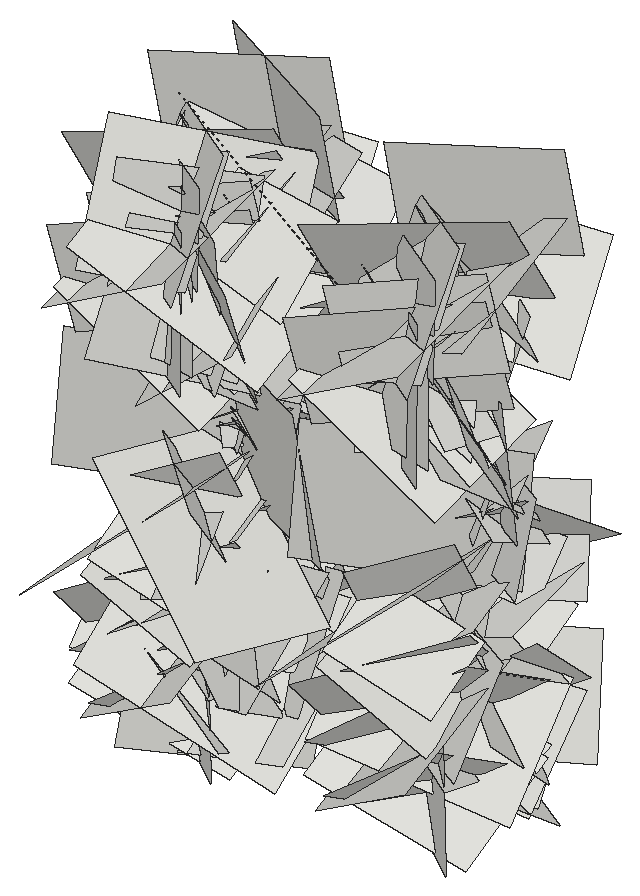
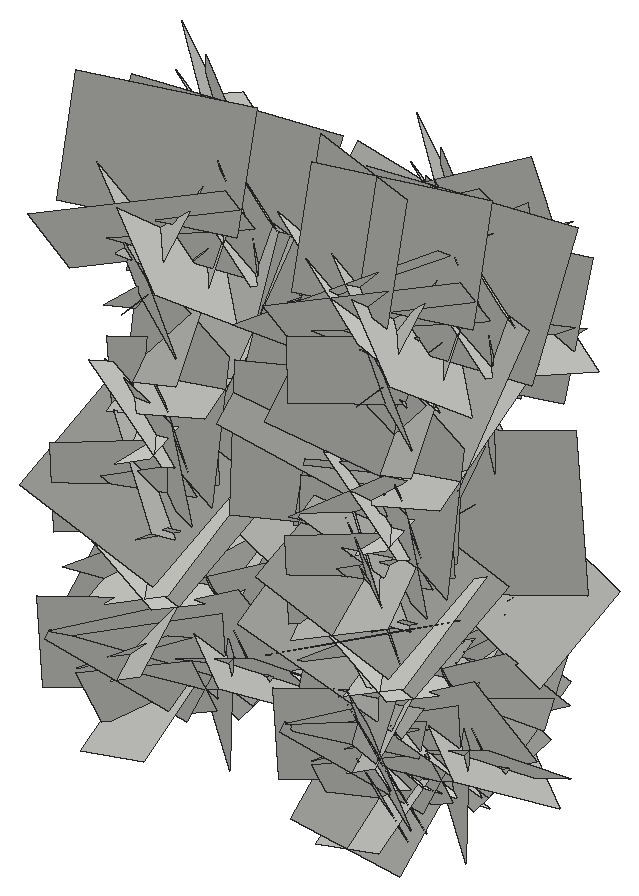
# SketchUp Ruby script. Lengths in inches.
U = 1.inch
M = Sketchup.active_model
def pt(a) = Geom::Point3d.new(a.map { |v| v * U })
def face(e, loops, mat)
  f = e.add_face(loops[0].map { |a| pt(a) })
  loops[1..].each { |l| e.add_face(l.map { |a| pt(a) }).erase! }
  f.material = f.back_material = mat if mat
  f
end
# faces: each face lists its corners as indices into pts; further lists are holes
def faces(e, pts, list, mat = nil) = list.each { |f| face(e, (f[0].is_a?(Array) ? f : [f]).map { |l| l.map { |i| pts[i] } }, mat) }
# xy, xz, yz: faces in a plane at the given z, y or x. An outline is a flat list of corners, or four numbers for a rectangle; further outlines are holes
def ring(l) = l.size == 4 ? [[l[0], l[1]], [l[2], l[1]], [l[2], l[3]], [l[0], l[3]]] : l.each_slice(2).to_a
def flat(e, list, mat, &to3) = list.each { |f| face(e, (f[0].is_a?(Array) ? f : [f]).map { |l| ring(l).map { |u, v| to3.(u, v) } }, mat) }
def xy(e, z, list, mat = nil) = flat(e, list, mat) { |x, y| [x, y, z] }
def xz(e, y, list, mat = nil) = flat(e, list, mat) { |x, z| [x, y, z] }
def yz(e, x, list, mat = nil) = flat(e, list, mat) { |y, z| [x, y, z] }
def lines(e, pts, list) = list.each { |a, b| e.add_line(pt(pts[a]), pt(pts[b])) }
# prism: a flat outline (further loops are holes) pulled along v
def prism(e, loops, v, mat = nil)
  f = face(e, loops, mat); d = Geom::Vector3d.new(v.map { |x| x * U })
  f.pushpull(f.normal.samedirection?(d) ? d.length : -d.length)
end
def box(e, o, s, mat = nil) = prism(e, [[o, [o[0] + s[0], o[1], o[2]], [o[0] + s[0], o[1] + s[1], o[2]], [o[0], o[1] + s[1], o[2]]]], [0, 0, s[2]], mat)
def at(x, y, z, deg = 0) = Geom::Transformation.translation(pt([x, y, z])) * Geom::Transformation.rotation(ORIGIN, Z_AXIS, deg.degrees)
def axes(o, x, y, z) = Geom::Transformation.new([*x, 0, *y, 0, *z, 0, *pt(o).to_a, 1])
def part(name) = M.definitions.add(name)
# library, detail: a bought-in or finely detailed component or shape, given as its bounding box
def library(name, o, s) = part(name).tap { |d| box(d.entities, o, s) }
def detail(e, o, s) = box(e.add_group.entities, o, s)
def put(e, d, t, mat = nil) = e.add_instance(d, t).tap { |i| i.material = mat if mat }
def group(e, t, mat = nil) = e.add_group.tap { |g| g.transformation = t; g.material = mat if mat }.entities
root = M.entities
c1 = part("Component\#6")
p = [[0.01,0,0],[0,3.24,4.54],[4.32,3.24,4.54],[4.33,0,0]]
faces(c1.entities,p,[[0,1,2,3]])
put(root,c1,axes([404.88,204.41,7.91],[-0.10208,-0.52254,-0.48763],[-0.08086,-0.48171,0.53127],[-0.75328,0.12252,0.00905]))
put(root,c1,axes([400.91,204.41,7.91],[0.10208,-0.52254,-0.48763],[0.08086,-0.48171,0.53127],[0.75328,0.12252,0.00905]))
put(root,c1,axes([414.68,204.41,7.91],[-0.10208,-0.52254,-0.48763],[-0.08086,-0.48171,0.53127],[-0.75328,0.12252,0.00905]))
put(root,c1,axes([400.91,200.61,7.25],[-0.15258,0.77944,0.1154],[-0.02035,0.1138,-0.79262],[0.83497,0.14521,0.00177]))
put(root,c1,axes([404.88,200.61,7.25],[0.15258,0.77944,0.1154],[0.02035,0.1138,-0.79262],[-0.83497,0.14521,0.00177]))
put(root,c1,axes([410.71,200.61,7.25],[-0.15258,0.77944,0.1154],[-0.02035,0.1138,-0.79262],[0.83497,0.14521,0.00177]))
put(root,c1,axes([404.88,201.43,15.61],[-0.13511,0.17275,0.7909],[-0.07376,0.79534,-0.18493],[-0.85494,-0.09592,-0.10904]))
put(root,c1,axes([400.91,201.43,15.61],[0.13511,0.17275,0.7909],[0.07376,0.79534,-0.18493],[0.85494,-0.09592,-0.10904]))
put(root,c1,axes([414.68,201.43,15.61],[-0.13511,0.17275,0.7909],[-0.07376,0.79534,-0.18493],[-0.85494,-0.09592,-0.10904]))
put(root,c1,axes([404.88,201.2,11.35],[-0.2643,1.29708,-0.17492],[0.19217,-0.14212,-1.31229],[-1.37397,-0.26938,-0.1499]))
put(root,c1,axes([400.91,201.2,11.35],[0.2643,1.29708,-0.17492],[-0.19217,-0.14212,-1.31229],[1.37397,-0.26938,-0.1499]))
put(root,c1,axes([414.68,201.2,11.35],[-0.2643,1.29708,-0.17492],[0.19217,-0.14212,-1.31229],[-1.37397,-0.26938,-0.1499]))
put(root,c1,axes([404.88,201.6875,18.6875],[-0.06388,0.10125,0.82658],[0.05301,0.82768,-0.09774],[-0.88113,0.04245,-0.0658]))
put(root,c1,axes([400.91,201.6875,18.6875],[0.06388,0.10125,0.82658],[-0.05301,0.82768,-0.09774],[0.88113,0.04245,-0.0658]))
put(root,c1,axes([414.68,201.6875,18.6875],[-0.06388,0.10125,0.82658],[0.05301,0.82768,-0.09774],[-0.88113,0.04245,-0.0658]))
put(root,c1,axes([404.88,204.39,20.61],[-0.01972,0.37325,-1.09096],[-0.03348,-1.09086,-0.37268],[-1.22177,0.02387,0.02782]))
put(root,c1,axes([400.91,204.39,20.61],[0.01972,0.37325,-1.09096],[0.03348,-1.09086,-0.37268],[1.22177,0.02387,0.02782]))
put(root,c1,axes([414.68,204.39,20.61],[-0.01972,0.37325,-1.09096],[-0.03348,-1.09086,-0.37268],[-1.22177,0.02387,0.02782]))
put(root,c1,axes([404.88,199.86,19.8],[0.08167,1.25653,0.46028],[-0.00634,0.46136,-1.25848],[-1.41846,0.07029,0.03212]))
put(root,c1,axes([400.91,199.86,19.8],[-0.08167,1.25653,0.46028],[0.00634,0.46136,-1.25848],[1.41846,0.07029,0.03212]))
put(root,c1,axes([414.68,199.86,19.8],[0.08167,1.25653,0.46028],[-0.00634,0.46136,-1.25848],[-1.41846,0.07029,0.03212]))
put(root,c1,axes([400.91,203.18,8],[0.06036,-0.35202,0.5516],[-0.07606,0.54699,0.35648],[0.68943,0.09116,-0.00896]))
put(root,c1,axes([404.88,203.18,8],[-0.06036,-0.35202,0.5516],[0.07606,0.54699,0.35648],[-0.68943,0.09116,-0.00896]))
put(root,c1,axes([410.71,203.18,8],[0.06036,-0.35202,0.5516],[-0.07606,0.54699,0.35648],[0.68943,0.09116,-0.00896]))
put(root,c1,axes([404.88,204.45,21.63],[0.07523,0.18922,-0.91056],[-0.04715,-0.91147,-0.19287],[-0.98469,0.0581,-0.06033]))
put(root,c1,axes([400.91,204.45,21.63],[-0.07523,0.18922,-0.91056],[0.04715,-0.91147,-0.19287],[0.98469,0.0581,-0.06033]))
put(root,c1,axes([414.68,204.45,21.63],[0.07523,0.18922,-0.91056],[-0.04715,-0.91147,-0.19287],[-0.98469,0.0581,-0.06033]))
put(root,c1,axes([404.88,203.64,8.5],[-0.20575,0.76434,-0.74551],[0.06488,-0.74852,-0.78336],[-1.12991,-0.18216,0.09078]))
put(root,c1,axes([400.91,203.64,8.5],[0.20575,0.76434,-0.74551],[-0.06488,-0.74852,-0.78336],[1.12991,-0.18216,0.09078]))
put(root,c1,axes([414.68,203.64,8.5],[-0.20575,0.76434,-0.74551],[0.06488,-0.74852,-0.78336],[-1.12991,-0.18216,0.09078]))
put(root,c1,axes([404.88,201.07,18.92],[-0.13602,0.69446,0.8684],[-0.06726,0.86816,-0.70365],[-1.17673,-0.1299,-0.06016]))
put(root,c1,axes([400.91,201.07,18.92],[0.13602,0.69446,0.8684],[0.06726,0.86816,-0.70365],[1.17673,-0.1299,-0.06016]))
put(root,c1,axes([414.68,201.07,18.92],[-0.13602,0.69446,0.8684],[-0.06726,0.86816,-0.70365],[-1.17673,-0.1299,-0.06016]))
put(root,c1,axes([404.88,200.34,18.7],[0.08817,0.51183,1.11442],[0.20058,1.09825,-0.51853],[-1.28435,0.20665,-0.00447]))
put(root,c1,axes([400.91,200.34,18.7],[-0.08817,0.51183,1.11442],[-0.20058,1.09825,-0.51853],[1.28435,0.20665,-0.00447]))
put(root,c1,axes([414.68,200.34,18.7],[0.08817,0.51183,1.11442],[0.20058,1.09825,-0.51853],[-1.28435,0.20665,-0.00447]))
put(root,c1,axes([404.88,200.79,15.19],[-0.21334,0.28139,1.2169],[0.22593,1.22225,-0.24738],[-1.30453,0.16566,-0.24185]))
put(root,c1,axes([400.91,200.79,15.19],[0.21334,0.28139,1.2169],[-0.22593,1.22225,-0.24738],[1.30453,0.16566,-0.24185]))
put(root,c1,axes([414.68,200.79,15.19],[-0.21334,0.28139,1.2169],[0.22593,1.22225,-0.24738],[-1.30453,0.16566,-0.24185]))
put(root,c1,axes([400.91,205.06,0.06],[-0.16762,-0.72435,0.3647],[-0.00744,0.37278,0.73735],[0.85961,-0.13802,0.0775]))
put(root,c1,axes([404.88,205.06,0.06],[0.16762,-0.72435,0.3647],[0.00744,0.37278,0.73735],[-0.85961,-0.13802,0.0775]))
put(root,c1,axes([410.71,205.06,0.06],[-0.16762,-0.72435,0.3647],[-0.00744,0.37278,0.73735],[0.85961,-0.13802,0.0775]))
put(root,c1,axes([400.91,202.62,14.39],[-0.09007,0.1944,0.61889],[0.03503,0.62466,-0.19168],[0.68673,-0.00637,0.09095]))
put(root,c1,axes([404.88,202.62,14.39],[0.09007,0.1944,0.61889],[-0.03503,0.62466,-0.19168],[-0.68673,-0.00637,0.09095]))
put(root,c1,axes([410.71,202.62,14.39],[-0.09007,0.1944,0.61889],[0.03503,0.62466,-0.19168],[0.68673,-0.00637,0.09095]))
put(root,c1,axes([404.88,200.25,4.04],[0.10038,1.14624,0.70824],[0.13093,0.69961,-1.1488],[-1.42222,0.14531,-0.05578]))
put(root,c1,axes([400.91,200.25,4.04],[-0.10038,1.14624,0.70824],[-0.13093,0.69961,-1.1488],[1.42222,0.14531,-0.05578]))
put(root,c1,axes([414.68,200.25,4.04],[0.10038,1.14624,0.70824],[0.13093,0.69961,-1.1488],[-1.42222,0.14531,-0.05578]))
put(root,c1,axes([404.88,207.09,15.04],[-0.15807,-1.02909,-0.4958],[0.14338,-0.5124,1.02286],[-1.20232,0.07419,0.18716]))
put(root,c1,axes([400.91,207.09,15.04],[0.15807,-1.02909,-0.4958],[-0.14338,-0.5124,1.02286],[1.20232,0.07419,0.18716]))
put(root,c1,axes([414.68,207.09,15.04],[-0.15807,-1.02909,-0.4958],[0.14338,-0.5124,1.02286],[-1.20232,0.07419,0.18716]))
put(root,c1,axes([400.91,205.68,16.84],[0.07036,-0.63328,-0.02287],[-0.09357,-0.03201,0.6302],[0.66517,0.06248,0.09107]))
put(root,c1,axes([404.88,205.68,16.84],[-0.07036,-0.63328,-0.02287],[0.09357,-0.03201,0.6302],[-0.66517,0.06248,0.09107]))
put(root,c1,axes([410.71,205.68,16.84],[0.07036,-0.63328,-0.02287],[-0.09357,-0.03201,0.6302],[0.66517,0.06248,0.09107]))
put(root,c1,axes([400.91,203.04,6.2],[-0.19197,0.78573,-0.28472],[-0.09491,-0.3079,-0.79273],[0.88077,0.13807,-0.14748]))
put(root,c1,axes([404.88,203.04,6.2],[0.19197,0.78573,-0.28472],[0.09491,-0.3079,-0.79273],[-0.88077,0.13807,-0.14748]))
put(root,c1,axes([410.71,203.04,6.2],[-0.19197,0.78573,-0.28472],[-0.09491,-0.3079,-0.79273],[0.88077,0.13807,-0.14748]))
put(root,c1,axes([404.88,203.52,7.375],[-0.0121,1.00291,-0.55649],[0.12117,-0.55275,-0.99852],[-1.20972,-0.0654,-0.09445]))
put(root,c1,axes([400.91,203.52,7.375],[0.0121,1.00291,-0.55649],[-0.12117,-0.55275,-0.99852],[1.20972,-0.0654,-0.09445]))
put(root,c1,axes([414.68,203.52,7.375],[-0.0121,1.00291,-0.55649],[0.12117,-0.55275,-0.99852],[-1.20972,-0.0654,-0.09445]))
put(root,c1,axes([404.88,202.39,0.06],[-0.12593,0.12266,1.10922],[0.15067,1.10807,-0.10731],[-1.17331,0.12913,-0.13284]))
put(root,c1,axes([400.91,202.39,0.06],[0.12593,0.12266,1.10922],[-0.15067,1.10807,-0.10731],[1.17331,0.12913,-0.13284]))
put(root,c1,axes([414.68,202.39,0.06],[-0.12593,0.12266,1.10922],[0.15067,1.10807,-0.10731],[-1.17331,0.12913,-0.13284]))
put(root,c1,axes([404.88,202.81,3.34],[0.17899,0.36268,0.93898],[-0.06935,0.95405,-0.35673],[-1.06473,-0.00117,0.18108]))
put(root,c1,axes([400.91,202.81,3.34],[-0.17899,0.36268,0.93898],[0.06935,0.95405,-0.35673],[1.06473,-0.00117,0.18108]))
put(root,c1,axes([414.68,202.81,3.34],[0.17899,0.36268,0.93898],[-0.06935,0.95405,-0.35673],[-1.06473,-0.00117,0.18108]))
put(root,c1,axes([404.88,203.75,8.58],[-0.14047,0.70659,0.15459],[0.00867,0.15861,-0.71798],[-0.76665,-0.12767,-0.03644]))
put(root,c1,axes([400.91,203.75,8.58],[0.14047,0.70659,0.15459],[-0.00867,0.15861,-0.71798],[0.76665,-0.12767,-0.03644]))
put(root,c1,axes([414.68,203.75,8.58],[-0.14047,0.70659,0.15459],[0.00867,0.15861,-0.71798],[-0.76665,-0.12767,-0.03644]))
put(root,c1,axes([404.88,206.9375,13.83],[-0.19711,0.10382,-1.30915],[-0.13395,-1.31749,-0.08653],[-1.38559,0.11259,0.1946]))
put(root,c1,axes([400.91,206.9375,13.83],[0.19711,0.10382,-1.30915],[0.13395,-1.31749,-0.08653],[1.38559,0.11259,0.1946]))
put(root,c1,axes([414.68,206.9375,13.83],[-0.19711,0.10382,-1.30915],[-0.13395,-1.31749,-0.08653],[-1.38559,0.11259,0.1946]))
put(root,c1,axes([404.88,207.71,2.15],[-0.07423,-0.90085,-0.6111],[-0.34403,-0.56723,0.87337],[-1.1014,0.23789,-0.23162]))
put(root,c1,axes([400.91,207.71,2.15],[0.07423,-0.90085,-0.6111],[0.34403,-0.56723,0.87337],[1.1014,0.23789,-0.23162]))
put(root,c1,axes([414.68,207.71,2.15],[-0.07423,-0.90085,-0.6111],[-0.34403,-0.56723,0.87337],[-1.1014,0.23789,-0.23162]))
put(root,c1,axes([400.91,204.05,18.57],[0.06151,0.80519,-0.14469],[-0.18353,-0.12968,-0.7911],[0.84753,-0.08652,-0.16081]))
put(root,c1,axes([404.88,204.05,18.57],[-0.06151,0.80519,-0.14469],[0.18353,-0.12968,-0.7911],[-0.84753,-0.08652,-0.16081]))
put(root,c1,axes([410.71,204.05,18.57],[0.06151,0.80519,-0.14469],[-0.18353,-0.12968,-0.7911],[0.84753,-0.08652,-0.16081]))
put(root,c1,axes([404.88,209.01,4.56],[0.09462,-0.88739,-0.86898],[-0.02241,-0.87218,0.88849],[-1.31634,-0.04894,-0.07759]))
put(root,c1,axes([400.91,209.01,4.56],[-0.09462,-0.88739,-0.86898],[0.02241,-0.87218,0.88849],[1.31634,-0.04894,-0.07759]))
put(root,c1,axes([414.68,209.01,4.56],[0.09462,-0.88739,-0.86898],[-0.02241,-0.87218,0.88849],[-1.31634,-0.04894,-0.07759]))
put(root,c1,axes([400.91,205.78,22.17],[0.00372,0.37911,-0.54343],[0.01311,-0.54338,-0.37899],[0.70223,0.00813,0.00995]))
put(root,c1,axes([404.88,205.78,22.17],[-0.00372,0.37911,-0.54343],[-0.01311,-0.54338,-0.37899],[-0.70223,0.00813,0.00995]))
put(root,c1,axes([410.71,205.78,22.17],[0.00372,0.37911,-0.54343],[0.01311,-0.54338,-0.37899],[0.70223,0.00813,0.00995]))
put(root,c1,axes([404.88,205.65,23.04],[-0.12198,0.70336,-1.01008],[-0.22842,-1.01033,-0.67899],[-1.28455,0.11286,0.21665]))
put(root,c1,axes([400.91,205.65,23.04],[0.12198,0.70336,-1.01008],[0.22842,-1.01033,-0.67899],[1.28455,0.11286,0.21665]))
put(root,c1,axes([414.68,205.65,23.04],[-0.12198,0.70336,-1.01008],[-0.22842,-1.01033,-0.67899],[-1.28455,0.11286,0.21665]))
put(root,c1,axes([404.88,205.49,13.28],[-0.13832,-0.68419,1.12815],[-0.08396,1.13567,0.67959],[-1.39605,-0.00051,-0.15265]))
put(root,c1,axes([400.91,205.49,13.28],[0.13832,-0.68419,1.12815],[0.08396,1.13567,0.67959],[1.39605,-0.00051,-0.15265]))
put(root,c1,axes([414.68,205.49,13.28],[-0.13832,-0.68419,1.12815],[-0.08396,1.13567,0.67959],[-1.39605,-0.00051,-0.15265]))
put(root,c1,axes([404.88,206.11,11.76],[0.09648,-0.72051,0.9522],[0.19874,0.95174,0.70224],[-1.25002,0.0957,0.18514]))
put(root,c1,axes([400.91,206.11,11.76],[-0.09648,-0.72051,0.9522],[-0.19874,0.95174,0.70224],[1.25002,0.0957,0.18514]))
put(root,c1,axes([414.68,206.11,11.76],[0.09648,-0.72051,0.9522],[0.19874,0.95174,0.70224],[-1.25002,0.0957,0.18514]))
put(root,c1,axes([404.88,207.28,11.15],[-0.07738,-1.09853,0.81062],[-0.01823,0.81245,1.09947],[-1.44703,0.04851,-0.0572]))
put(root,c1,axes([400.91,207.28,11.15],[0.07738,-1.09853,0.81062],[0.01823,0.81245,1.09947],[1.44703,0.04851,-0.0572]))
put(root,c1,axes([414.68,207.28,11.15],[-0.07738,-1.09853,0.81062],[-0.01823,0.81245,1.09947],[-1.44703,0.04851,-0.0572]))
put(root,c1,axes([404.88,207.17,17.14],[-0.0563,-0.55845,0.63654],[-0.00808,0.63808,0.55916],[-0.89756,0.02928,-0.04497]))
put(root,c1,axes([400.91,207.17,17.14],[0.0563,-0.55845,0.63654],[0.00808,0.63808,0.55916],[0.89756,0.02928,-0.04497]))
put(root,c1,axes([414.68,207.17,17.14],[-0.0563,-0.55845,0.63654],[-0.00808,0.63808,0.55916],[-0.89756,0.02928,-0.04497]))
put(root,c1,axes([404.88,203.17,19.17],[0.16233,1.06667,0.75788],[0.09967,0.75211,-1.07754],[-1.38342,0.17935,0.0113]))
put(root,c1,axes([400.91,203.17,19.17],[-0.16233,1.06667,0.75788],[-0.09967,0.75211,-1.07754],[1.38342,0.17935,0.0113]))
put(root,c1,axes([414.68,203.17,19.17],[0.16233,1.06667,0.75788],[0.09967,0.75211,-1.07754],[-1.38342,0.17935,0.0113]))
put(root,c1,axes([404.88,209.96,4.13],[-0.07876,-0.66244,-0.94852],[-0.03994,-0.94858,0.66543],[-1.2257,0.07348,0.03927]))
put(root,c1,axes([400.91,209.96,4.13],[0.07876,-0.66244,-0.94852],[0.03994,-0.94858,0.66543],[1.2257,0.07348,0.03927]))
put(root,c1,axes([414.68,209.96,4.13],[-0.07876,-0.66244,-0.94852],[-0.03994,-0.94858,0.66543],[-1.2257,0.07348,0.03927]))
put(root,c1,axes([400.91,209.54,8.98],[0.01886,-0.65319,-0.4186],[-0.2021,-0.40955,0.63097],[0.79714,-0.08839,0.16987]))
put(root,c1,axes([404.88,209.54,8.98],[-0.01886,-0.65319,-0.4186],[0.2021,-0.40955,0.63097],[-0.79714,-0.08839,0.16987]))
put(root,c1,axes([410.71,209.54,8.98],[0.01886,-0.65319,-0.4186],[-0.2021,-0.40955,0.63097],[0.79714,-0.08839,0.16987]))
put(root,c1,axes([400.91,205.65,3.3125],[0.06993,0.62057,0.27964],[0.0119,0.27992,-0.62384],[0.72141,-0.06477,-0.01682]))
put(root,c1,axes([404.88,205.65,3.3125],[-0.06993,0.62057,0.27964],[-0.0119,0.27992,-0.62384],[-0.72141,-0.06477,-0.01682]))
put(root,c1,axes([410.71,205.65,3.3125],[0.06993,0.62057,0.27964],[0.0119,0.27992,-0.62384],[0.72141,-0.06477,-0.01682]))
put(root,c1,axes([400.91,208.89,13.53],[-0.18208,-0.09561,-0.67164],[-0.05748,-0.68868,0.1119],[0.71681,-0.07951,-0.16163]))
put(root,c1,axes([404.88,208.89,13.53],[0.18208,-0.09561,-0.67164],[0.05748,-0.68868,0.1119],[-0.71681,-0.07951,-0.16163]))
put(root,c1,axes([410.71,208.89,13.53],[-0.18208,-0.09561,-0.67164],[-0.05748,-0.68868,0.1119],[0.71681,-0.07951,-0.16163]))
put(root,c1,axes([404.88,205.98,8.7],[0.1184,0.10295,0.88925],[-0.12891,0.88959,-0.08771],[-0.94011,-0.10902,0.12403]))
put(root,c1,axes([400.91,205.98,8.7],[-0.1184,0.10295,0.88925],[0.12891,0.88959,-0.08771],[0.94011,-0.10902,0.12403]))
put(root,c1,axes([414.68,205.98,8.7],[0.1184,0.10295,0.88925],[-0.12891,0.88959,-0.08771],[-0.94011,-0.10902,0.12403]))
put(root,c1,axes([400.91,207.72,1.15],[-0.00392,-0.70388,0.63123],[-0.16138,0.62344,0.69431],[0.98911,0.09893,0.11578]))
put(root,c1,axes([404.88,207.72,1.15],[0.00392,-0.70388,0.63123],[0.16138,0.62344,0.69431],[-0.98911,0.09893,0.11578]))
put(root,c1,axes([410.71,207.72,1.15],[-0.00392,-0.70388,0.63123],[-0.16138,0.62344,0.69431],[0.98911,0.09893,0.11578]))
put(root,c1,axes([414.68,207.72,1.15],[0.00392,-0.70388,0.63123],[0.16138,0.62344,0.69431],[-0.98911,0.09893,0.11578]))
put(root,c1,axes([404.88,208.78,4.43],[-0.01106,-0.99025,0.53374],[-0.00744,0.53381,0.99025],[-1.19241,0.00586,-0.01113]))
put(root,c1,axes([400.91,208.78,4.43],[0.01106,-0.99025,0.53374],[0.00744,0.53381,0.99025],[1.19241,0.00586,-0.01113]))
put(root,c1,axes([414.68,208.78,4.43],[-0.01106,-0.99025,0.53374],[-0.00744,0.53381,0.99025],[-1.19241,0.00586,-0.01113]))
put(root,c1,axes([400.91,206.67,12.85],[0.04142,0.63331,-0.27554],[0.00251,-0.27611,-0.63426],[0.73209,-0.03488,0.01776]))
put(root,c1,axes([404.88,206.67,12.85],[-0.04142,0.63331,-0.27554],[-0.00251,-0.27611,-0.63426],[-0.73209,-0.03488,0.01776]))
put(root,c1,axes([410.71,206.67,12.85],[0.04142,0.63331,-0.27554],[0.00251,-0.27611,-0.63426],[0.73209,-0.03488,0.01776]))
put(root,c1,axes([404.88,206.09,10.75],[-0.05447,-0.13377,1.26127],[-0.13355,1.2566,0.12815],[-1.33779,-0.12,-0.06414]))
put(root,c1,axes([400.91,206.09,10.75],[0.05447,-0.13377,1.26127],[0.13355,1.2566,0.12815],[1.33779,-0.12,-0.06414]))
put(root,c1,axes([414.68,206.09,10.75],[-0.05447,-0.13377,1.26127],[-0.13355,1.2566,0.12815],[-1.33779,-0.12,-0.06414]))
put(root,c1,axes([404.88,206,12.43],[-0.16769,0.64159,0.3622],[0.01184,0.3725,-0.65496],[-0.78088,-0.13213,-0.08771]))
put(root,c1,axes([400.91,206,12.43],[0.16769,0.64159,0.3622],[-0.01184,0.3725,-0.65496],[0.78088,-0.13213,-0.08771]))
put(root,c1,axes([414.68,206,12.43],[-0.16769,0.64159,0.3622],[0.01184,0.3725,-0.65496],[-0.78088,-0.13213,-0.08771]))
put(root,c1,axes([400.91,206.15,0.87],[-0.01906,0.33732,0.58365],[0.0637,0.58234,-0.33471],[0.71172,-0.04309,0.04558]))
put(root,c1,axes([404.88,206.15,0.87],[0.01906,0.33732,0.58365],[-0.0637,0.58234,-0.33471],[-0.71172,-0.04309,0.04558]))
put(root,c1,axes([410.71,206.15,0.87],[-0.01906,0.33732,0.58365],[0.0637,0.58234,-0.33471],[0.71172,-0.04309,0.04558]))
put(root,c1,axes([404.88,208.53,24.44],[-0.00063,0.23668,-1.01361],[-0.18606,-0.99912,-0.23319],[-1.08753,0.17079,0.04049]))
put(root,c1,axes([400.91,208.53,24.44],[0.00063,0.23668,-1.01361],[0.18606,-0.99912,-0.23319],[1.08753,0.17079,0.04049]))
put(root,c1,axes([414.68,208.53,24.44],[-0.00063,0.23668,-1.01361],[-0.18606,-0.99912,-0.23319],[-1.08753,0.17079,0.04049]))
put(root,c1,axes([404.88,206.6,8.35],[-0.07615,0.29672,0.54367],[-0.07213,0.54022,-0.30383],[-0.65256,-0.09434,-0.02986]))
put(root,c1,axes([400.91,206.6,8.35],[0.07615,0.29672,0.54367],[0.07213,0.54022,-0.30383],[0.65256,-0.09434,-0.02986]))
put(root,c1,axes([410.71,206.6,8.35],[0.07615,0.29672,0.54367],[0.07213,0.54022,-0.30383],[0.65256,-0.09434,-0.02986]))
put(root,c1,axes([404.88,211.08,20.1875],[0.1855,-0.74932,-0.85781],[-0.09412,-0.87421,0.74553],[-1.20366,-0.04712,-0.19049]))
put(root,c1,axes([400.91,211.08,20.1875],[-0.1855,-0.74932,-0.85781],[0.09412,-0.87421,0.74553],[1.20366,-0.04712,-0.19049]))
put(root,c1,axes([414.68,211.08,20.1875],[0.1855,-0.74932,-0.85781],[-0.09412,-0.87421,0.74553],[-1.20366,-0.04712,-0.19049]))
put(root,c1,axes([404.88,206.49,12.28],[0.17995,0.92169,-0.62911],[-0.1265,-0.6177,-0.93718],[-1.17609,0.20746,0.00455]))
put(root,c1,axes([400.91,206.49,12.28],[-0.17995,0.92169,-0.62911],[0.1265,-0.6177,-0.93718],[1.17609,0.20746,0.00455]))
put(root,c1,axes([414.68,206.49,12.28],[0.17995,0.92169,-0.62911],[-0.1265,-0.6177,-0.93718],[-1.17609,0.20746,0.00455]))
put(root,c1,axes([400.91,206.02,7.14],[0.00935,0.6115,0.38278],[-0.02819,0.38283,-0.61096],[0.76419,0.00664,-0.02722]))
put(root,c1,axes([404.88,206.02,7.14],[-0.00935,0.6115,0.38278],[0.02819,0.38283,-0.61096],[-0.76419,0.00664,-0.02722]))
put(root,c1,axes([410.71,206.02,7.14],[0.00935,0.6115,0.38278],[-0.02819,0.38283,-0.61096],[0.76419,0.00664,-0.02722]))
put(root,c1,axes([400.91,207.38,2.3],[0.03327,0.56132,-0.40527],[0.08729,-0.40584,-0.55572],[0.72866,0.02299,0.08508]))
put(root,c1,axes([404.88,207.38,2.3],[-0.03327,0.56132,-0.40527],[-0.08729,-0.40584,-0.55572],[-0.72866,0.02299,0.08508]))
put(root,c1,axes([410.71,207.38,2.3],[0.03327,0.56132,-0.40527],[0.08729,-0.40584,-0.55572],[0.72866,0.02299,0.08508]))
put(root,c1,axes([404.88,205.78,7.5],[0.02909,0.83454,0.28231],[-0.13137,0.2833,-0.8254],[-0.92457,-0.01399,0.12617]))
put(root,c1,axes([400.91,205.78,7.5],[-0.02909,0.83454,0.28231],[0.13137,0.2833,-0.8254],[0.92457,-0.01399,0.12617]))
put(root,c1,axes([414.68,205.78,7.5],[0.02909,0.83454,0.28231],[-0.13137,0.2833,-0.8254],[-0.92457,-0.01399,0.12617]))
put(root,c1,axes([400.91,205.95,7.64],[-0.13368,0.21915,0.90835],[-0.05222,0.91375,-0.2273],[0.9891,0.07786,0.11076]))
put(root,c1,axes([404.88,205.95,7.64],[0.13368,0.21915,0.90835],[0.05222,0.91375,-0.2273],[-0.9891,0.07786,0.11076]))
put(root,c1,axes([410.71,205.95,7.64],[-0.13368,0.21915,0.90835],[-0.05222,0.91375,-0.2273],[0.9891,0.07786,0.11076]))
put(root,c1,axes([400.91,209.83,18.53],[-0.13516,-0.18826,-0.70807],[-0.00477,-0.7185,0.19184],[0.77662,-0.03718,-0.12206]))
put(root,c1,axes([404.88,209.83,18.53],[0.13516,-0.18826,-0.70807],[0.00477,-0.7185,0.19184],[-0.77662,-0.03718,-0.12206]))
put(root,c1,axes([410.71,209.83,18.53],[-0.13516,-0.18826,-0.70807],[-0.00477,-0.7185,0.19184],[0.77662,-0.03718,-0.12206]))
put(root,c1,axes([404.88,210.56,5.71],[0.17873,-0.295,-0.9769],[-0.02803,-0.99107,0.29472],[-1.08133,-0.02307,-0.16911]))
put(root,c1,axes([400.91,210.56,5.71],[-0.17873,-0.295,-0.9769],[0.02803,-0.99107,0.29472],[1.08133,-0.02307,-0.16911]))
put(root,c1,axes([414.68,210.56,5.71],[0.17873,-0.295,-0.9769],[-0.02803,-0.99107,0.29472],[-1.08133,-0.02307,-0.16911]))
put(root,c1,axes([400.91,208.64,6.82],[0.0498,0.28937,-0.67344],[0.06797,-0.67386,-0.28508],[0.77398,0.04056,0.06836]))
put(root,c1,axes([404.88,208.64,6.82],[-0.0498,0.28937,-0.67344],[-0.06797,-0.67386,-0.28508],[-0.77398,0.04056,0.06836]))
